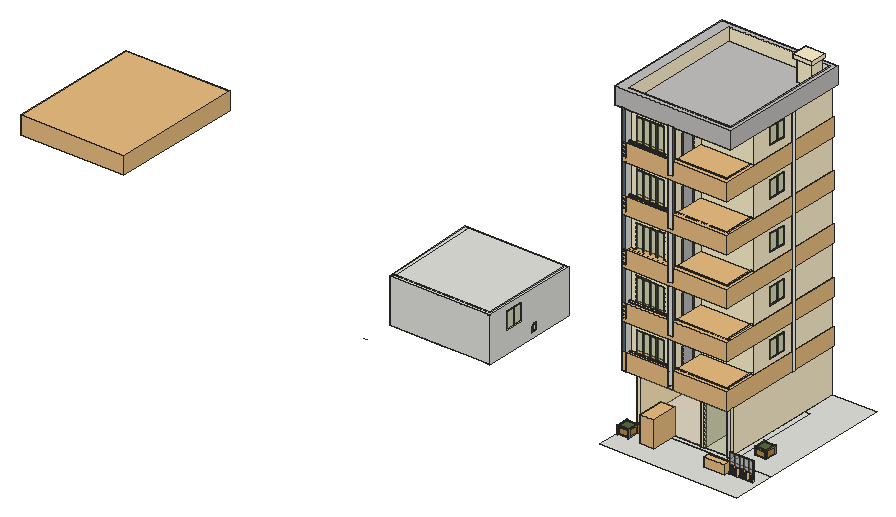
# SketchUp Ruby script. Lengths in inches.
U = 1.inch
M = Sketchup.active_model
def pt(a) = Geom::Point3d.new(a.map { |v| v * U })
def face(e, loops, mat)
  f = e.add_face(loops[0].map { |a| pt(a) })
  loops[1..].each { |l| e.add_face(l.map { |a| pt(a) }).erase! }
  f.material = f.back_material = mat if mat
  f
end
# faces: each face lists its corners as indices into pts; further lists are holes
def faces(e, pts, list, mat = nil) = list.each { |f| face(e, (f[0].is_a?(Array) ? f : [f]).map { |l| l.map { |i| pts[i] } }, mat) }
# xy, xz, yz: faces in a plane at the given z, y or x. An outline is a flat list of corners, or four numbers for a rectangle; further outlines are holes
def ring(l) = l.size == 4 ? [[l[0], l[1]], [l[2], l[1]], [l[2], l[3]], [l[0], l[3]]] : l.each_slice(2).to_a
def flat(e, list, mat, &to3) = list.each { |f| face(e, (f[0].is_a?(Array) ? f : [f]).map { |l| ring(l).map { |u, v| to3.(u, v) } }, mat) }
def xy(e, z, list, mat = nil) = flat(e, list, mat) { |x, y| [x, y, z] }
def xz(e, y, list, mat = nil) = flat(e, list, mat) { |x, z| [x, y, z] }
def yz(e, x, list, mat = nil) = flat(e, list, mat) { |y, z| [x, y, z] }
def lines(e, pts, list) = list.each { |a, b| e.add_line(pt(pts[a]), pt(pts[b])) }
# prism: a flat outline (further loops are holes) pulled along v
def prism(e, loops, v, mat = nil)
  f = face(e, loops, mat); d = Geom::Vector3d.new(v.map { |x| x * U })
  f.pushpull(f.normal.samedirection?(d) ? d.length : -d.length)
end
def box(e, o, s, mat = nil) = prism(e, [[o, [o[0] + s[0], o[1], o[2]], [o[0] + s[0], o[1] + s[1], o[2]], [o[0], o[1] + s[1], o[2]]]], [0, 0, s[2]], mat)
def at(x, y, z, deg = 0) = Geom::Transformation.translation(pt([x, y, z])) * Geom::Transformation.rotation(ORIGIN, Z_AXIS, deg.degrees)
def axes(o, x, y, z) = Geom::Transformation.new([*x, 0, *y, 0, *z, 0, *pt(o).to_a, 1])
def part(name) = M.definitions.add(name)
# library, detail: a bought-in or finely detailed component or shape, given as its bounding box
def library(name, o, s) = part(name).tap { |d| box(d.entities, o, s) }
def detail(e, o, s) = box(e.add_group.entities, o, s)
def put(e, d, t, mat = nil) = e.add_instance(d, t).tap { |i| i.material = mat if mat }
def group(e, t, mat = nil) = e.add_group.tap { |g| g.transformation = t; g.material = mat if mat }.entities
root = M.entities
M.materials.add("!长灌木1").color = [90, 107, 61]
M.materials.add("Carpet_01_1K").color = [196, 195, 193]
M.materials.add("D01_Frost_White").color = [255, 242, 206]
M.materials.add("Denim_03_1K").color = [93, 106, 119]
M.materials.add("Glass_Basic_01").color = [179, 186, 71]
M.materials["Glass_Basic_01"].alpha = 0.25
M.materials.add("Glass_Basic_1").color = [255, 210, 130]
M.materials["Glass_Basic_1"].alpha = 0.25
M.materials.add("Glass_Mirror_01").color = [185, 185, 185]
M.materials.add("M00_Soft_Cloud").color = [255, 255, 255]
M.materials.add("Material20").color = [184, 138, 65]
M.materials.add("Material48").color = [126, 124, 110]
M.materials.add("Material__1").color = [95, 70, 46]
M.materials.add("Wood_Planks_01_1K").color = [69, 67, 63]
M.materials.add("[Color M00]").color = [255, 255, 255]
M.materials.add("[Translucent Glass Gray]").color = [128, 128, 128]
M.materials["[Translucent Glass Gray]"].alpha = 0.29
M.materials.add("homalw").color = [47, 64, 22]
M.materials.add("palmleaf1").color = [111, 131, 65]
c1 = library("Balcony with railing",[0,-15.52,0],[286.53,362.52,46.98])
c2 = part("Building bay")
xy(c2.entities,0,[[0,-15.52,12,0],[125.84,-15.52,138,0],[9,9,129,80],[9,89,273,338]])
xy(c2.entities,16.02,[[273,223.5625,282,234.47]])
xy(c2.entities,34.07,[[273,223.5625,282,234.47]])
xy(c2.entities,120,[[0,-15.52,9,347],[9,-15.52,12,-15.52,12,0,125.84,0,125.84,-15.52,138,-15.52,138,80.06,282,80.06,282,347,9,347,9,338,273,338,273,89,9,89,9,80,129,80,129,9,9,9],[9,89,273,338]])
xy(c2.entities,120,[[9,9,129,80]],"Denim_03_1K")
xz(c2.entities,-15.52,[[125.84,0,138,120]])
xz(c2.entities,-15.52,[[0,0,12,120]],"Denim_03_1K")
xz(c2.entities,0,[[[12,0,125.84,120],[26.96,12.98,106.4,103.84]]],"D01_Frost_White")
xz(c2.entities,0,[[29.96,15.98,45.32,100.84],[48.32,15.98,63.68,100.84],[66.68,15.98,82.04,100.84],[85.04,15.98,103.4,100.84]],"Glass_Basic_01")
xz(c2.entities,0,[[[26.96,12.98,106.4,103.84],[85.04,15.98,103.4,100.84],[48.32,15.98,63.68,100.84],[66.68,15.98,82.04,100.84],[29.96,15.98,45.32,100.84]]],"Wood_Planks_01_1K")
xz(c2.entities,9,[[9,0,129,120]])
xz(c2.entities,80,[[9,0,129,120]])
xz(c2.entities,80.06,[[138,0,282,120]],"D01_Frost_White")
xz(c2.entities,89,[[9,0,273,120]])
xz(c2.entities,223.5625,[[273,16.02,282,34.07]])
xz(c2.entities,234.47,[[273,16.02,282,34.07]])
xz(c2.entities,338,[[9,0,273,120]])
xz(c2.entities,347,[[0,0,282,120]])
yz(c2.entities,0,[[-15.52,0,347,120]],"D01_Frost_White")
yz(c2.entities,9,[[9,0,80,120],[89,0,338,120]])
yz(c2.entities,12,[[-15.52,0,0,120]])
yz(c2.entities,125.84,[[-15.52,0,0,120]])
yz(c2.entities,129,[[9,0,80,120]])
yz(c2.entities,138,[[-7.18,10,-7.09,120]])
yz(c2.entities,138,[[[-15.52,0,80.06,0,80.06,120,-7.09,120,-7.09,10,-15.52,10],[17.75,12.24,56.41,97.36]]],"D01_Frost_White")
yz(c2.entities,138,[[-15.52,10,-7.18,120]],"Denim_03_1K")
yz(c2.entities,138,[[20.75,15.24,53.41,94.36]],"Glass_Mirror_01")
yz(c2.entities,138,[[[17.75,12.24,56.41,97.36],[20.75,15.24,53.41,94.36]]],"Wood_Planks_01_1K")
yz(c2.entities,273,[[[89,0,338,120],[223.5625,16.02,234.47,34.07]]])
yz(c2.entities,282,[[[80.06,0,347,120],[133.09,55.97,187.08,106.98],[222.16,14.62,235.875,35.48]]],"D01_Frost_White")
yz(c2.entities,282,[[136.83,59.71,160.08,103.24],[163.08,59.71,183.34,103.24]],"Glass_Basic_01")
yz(c2.entities,282,[[[222.16,14.62,235.875,35.48],[223.5625,16.02,234.47,34.07]],[[133.09,55.97,187.08,106.98],[136.83,59.71,183.34,103.24]],[160.08,59.71,163.08,103.24]],"Wood_Planks_01_1K")
c3 = part("Flat roof assembly")
xy(c3.entities,-639.97,[[282,205.21,288.51,211.41]])
xy(c3.entities,-6.48,[[158.77,-7.18,158.77,211.41,282,211.41,282,205.21,288.51,205.21,288.51,-7.18],[282,211.41,282,211.54,293.15,211.41]])
xy(c3.entities,0,[[[-17.96,-15,297.5,347],[158.77,-7.18,288.51,211.41]]])
xy(c3.entities,10,[[[11.4,-3.6,286.1,335.6],[232.625,289.57,272.46,324.45]]],"Carpet_01_1K")
xy(c3.entities,46,[[[-17.96,-15,297.5,347],[11.4,-3.6,286.1,335.6]]],"Carpet_01_1K")
xy(c3.entities,66.73,[[[224.49,284,277.47,329.34],[232.625,289.57,272.46,324.45]],[232.625,289.57,272.46,324.45]])
xy(c3.entities,76.73,[[224.49,284,277.47,329.34]])
xz(c3.entities,-15,[[-17.96,0,297.5,46]],"Carpet_01_1K")
xz(c3.entities,-7.18,[[158.77,-6.48,288.51,0]])
xz(c3.entities,-3.6,[[11.4,10,12,46]])
xz(c3.entities,-3.6,[[12,10,125.84,46],[125.84,10,138,46],[138,10,286.1,46]],"Carpet_01_1K")
xz(c3.entities,205.21,[[282,-639.97,288.51,-6.48]])
xz(c3.entities,211.41,[[282,-639.97,288.51,-6.48],[158.77,-6.48,288.51,0]])
xz(c3.entities,284,[[224.49,66.73,277.47,76.73]])
xz(c3.entities,289.57,[[232.625,10,272.46,66.73]])
xz(c3.entities,324.45,[[232.625,10,272.46,66.73]])
xz(c3.entities,329.34,[[224.49,66.73,277.47,76.73]])
xz(c3.entities,335.6,[[11.4,10,286.1,46]])
xz(c3.entities,347,[[-17.96,0,297.5,46]],"Carpet_01_1K")
yz(c3.entities,-17.96,[[-15,0,347,46]],"Carpet_01_1K")
yz(c3.entities,11.4,[[-3.6,10,335.6,46]])
yz(c3.entities,158.77,[[-7.18,-6.48,211.41,0]])
yz(c3.entities,224.49,[[284,66.73,329.34,76.73]])
yz(c3.entities,232.625,[[289.57,10,324.45,66.73]])
yz(c3.entities,272.46,[[289.57,10,324.45,66.73]])
yz(c3.entities,277.47,[[284,66.73,329.34,76.73]])
yz(c3.entities,282,[[205.21,-639.97,211.41,-6.48]])
yz(c3.entities,286.1,[[-3.6,10,335.6,46]],"Carpet_01_1K")
yz(c3.entities,288.51,[[205.21,-639.97,211.41,-639.97,211.41,0,-7.18,0,-7.18,-6.48,205.21,-6.48]],"M00_Soft_Cloud")
yz(c3.entities,297.5,[[-15,0,347,46]],"Carpet_01_1K")
c4 = library("Balcony railing",[0,-12,0],[282,359,46.98])
c5 = part("组\#1")
xy(c5.entities,0,[[0,0,2.36,2.36],[29.92,0,32.28,2.36],[0,29.92,2.36,32.28],[29.92,29.92,32.28,32.28]],"Material48")
xy(c5.entities,1.57,[[2.36,0.39,2.36,2.36,0.39,2.36,0.39,29.92,2.36,29.92,2.36,31.89,29.92,31.89,29.92,29.92,31.89,29.92,31.89,2.36,29.92,2.36,29.92,0.39]],"Material48")
xy(c5.entities,2.76,[[3.54,0.39,28.74,1.57],[0.39,3.54,1.57,28.74],[30.71,3.54,31.89,28.74],[3.54,30.71,28.74,31.89]],"Material20")
xy(c5.entities,20.08,[[3.54,0.39,28.74,1.57],[0.39,3.54,1.57,28.74],[30.71,3.54,31.89,28.74],[3.54,30.71,28.74,31.89]],"Material20")
xy(c5.entities,21.0625,[[2.36,2.36,29.92,29.92]],"!长灌木1")
xy(c5.entities,21.26,[[2.36,0.39,29.92,2.36],[0.39,2.36,2.36,29.92],[29.92,2.36,31.89,29.92],[2.36,29.92,29.92,31.89]],"Material20")
xy(c5.entities,21.38,[[2.36,2.36,29.92,29.92]],"!长灌木1")
xy(c5.entities,22.83,[[0,0,2.36,2.36],[29.92,0,32.28,2.36],[0,29.92,2.36,32.28],[29.92,29.92,32.28,32.28]],"Material20")
xz(c5.entities,0,[[0,0,2.36,22.83],[29.92,0,32.28,22.83]],"Material20")
xz(c5.entities,0.39,[[[2.36,1.57,29.92,21.26],[3.54,2.76,28.74,20.08]]],"Material20")
xz(c5.entities,1.57,[[3.54,2.76,28.74,20.08]],"Material20")
xz(c5.entities,2.36,[[2.36,21.0625,29.92,21.38],[2.36,21.26,29.92,23.43]],"!长灌木1")
xz(c5.entities,2.36,[[0,0,0,22.83,2.36,22.83,2.36,21.26,0.39,21.26,0.39,1.57,2.36,1.57,2.36,0],[29.92,0,29.92,1.57,31.89,1.57,31.89,21.26,29.92,21.26,29.92,22.83,32.28,22.83,32.28,0]],"Material20")
xz(c5.entities,3.54,[[0.39,2.76,1.57,20.08],[30.71,2.76,31.89,20.08]],"Material20")
xz(c5.entities,28.74,[[0.39,2.76,1.57,20.08],[30.71,2.76,31.89,20.08]],"Material20")
xz(c5.entities,29.92,[[2.36,21.0625,29.92,21.38],[2.36,21.26,29.92,23.43]],"!长灌木1")
xz(c5.entities,29.92,[[0,0,2.36,0,2.36,1.57,0.39,1.57,0.39,22.83,0,22.83],[29.92,0,32.28,0,32.28,22.83,31.89,22.83,31.89,1.57,29.92,1.57],[0.39,21.26,2.36,22.83],[29.92,21.26,31.89,22.83]],"Material20")
xz(c5.entities,30.71,[[3.54,2.76,28.74,20.08]],"Material20")
xz(c5.entities,31.89,[[[2.36,1.57,29.92,21.26],[3.54,2.76,28.74,20.08]]],"Material20")
xz(c5.entities,32.28,[[0,0,2.36,22.83],[29.92,0,32.28,22.83]],"Material20")
yz(c5.entities,0,[[0,0,2.36,22.83],[29.92,0,32.28,22.83]],"Material20")
yz(c5.entities,0.39,[[[2.36,1.57,29.92,21.26],[3.54,2.76,28.74,20.08]]],"Material20")
yz(c5.entities,1.57,[[3.54,2.76,28.74,20.08]],"Material20")
yz(c5.entities,2.36,[[0,0,2.36,0,2.36,1.57,0.39,1.57,0.39,22.83,0,22.83]])
yz(c5.entities,2.36,[[2.36,21.0625,29.92,21.38],[2.36,21.26,29.92,23.43]],"!长灌木1")
yz(c5.entities,2.36,[[29.92,0,32.28,0,32.28,22.83,29.92,22.83,29.92,21.26,31.89,21.26,31.89,1.57,29.92,1.57],[0.39,21.26,2.36,22.83]],"Material20")
yz(c5.entities,3.54,[[0.39,2.76,1.57,20.08],[30.71,2.76,31.89,20.08]],"Material20")
yz(c5.entities,28.74,[[0.39,2.76,1.57,20.08],[30.71,2.76,31.89,20.08]],"Material20")
yz(c5.entities,29.92,[[2.36,21.0625,29.92,21.38],[2.36,21.26,29.92,23.43]],"!长灌木1")
yz(c5.entities,29.92,[[0,0,0,22.83,2.36,22.83,2.36,21.26,0.39,21.26,0.39,1.57,2.36,1.57,2.36,0],[29.92,0,29.92,1.57,31.89,1.57,31.89,21.26,29.92,21.26,29.92,22.83,32.28,22.83,32.28,0]],"Material20")
yz(c5.entities,30.71,[[3.54,2.76,28.74,20.08]],"Material20")
yz(c5.entities,31.89,[[[2.36,1.57,29.92,21.26],[3.54,2.76,28.74,20.08]]],"Material20")
yz(c5.entities,32.28,[[0,0,2.36,22.83],[29.92,0,32.28,22.83]],"Material20")
c6 = part("组\#2")
put(c6.entities,c5,at(24.1,23.99,0))
c7 = part("Tree in planter")
put(c7.entities,c6,at(-24.1,-23.99,-1.57))
c8 = library("Planted timber trough",[0,0,0],[56.02,15.3,25.28])
c9 = library("Group_2",[-1.28,-0.39,0],[21.22,20.51,48.44])
c10 = library("Areca palm plant",[0,0,0],[49.1,36.6,54.46])
c11 = part("W1")
xy(c11.entities,15,[[0,0,2,198]])
xy(c11.entities,102.0625,[[0,0,2,198]],"[Color M00]")
xz(c11.entities,0,[[0,15,2,102.0625]],"[Color M00]")
xz(c11.entities,198,[[0,15,2,102.0625]])
yz(c11.entities,0,[[0.84,16,39.43,101.0625],[40.28,16,78.87,101.0625],[79.71,16,118.3,101.0625],[119.14,16,157.73,101.0625],[158.58,16,197.16,101.0625]])
yz(c11.entities,0,[[[0,15,198,102.0625],[0.84,16,197.16,101.0625]],[39.43,16,40.28,101.0625],[78.87,16,79.71,101.0625],[118.3,16,119.14,101.0625],[157.73,16,158.58,101.0625]],"[Color M00]")
yz(c11.entities,2,[[0.84,16,39.43,101.0625],[40.28,16,78.87,101.0625],[79.71,16,118.3,101.0625],[119.14,16,157.73,101.0625],[158.58,16,197.16,101.0625]])
yz(c11.entities,2,[[[0,15,198,102.0625],[0.84,16,197.16,101.0625]],[39.43,16,40.28,101.0625],[78.87,16,79.71,101.0625],[118.3,16,119.14,101.0625],[157.73,16,158.58,101.0625]],"[Color M00]")
c12 = part("Leaf \#1")
xy(c12.entities,0,[[-7.96,70.18,-15.37,80.78,-8.51,79.39]],"homalw")
p = [[0,3.11,-13.12],[-2.47,2.5625,-12.61],[-0.33,11.57,-7.99],[2.47,2.5625,-12.61],[0.85,11.07,-7.46],[-1.5,10.97,-7.51],
  [-1.3,12.65,-6.5],[0.75,12.74,-6.45],[-0.28,13.24,-6.98],[-0.52,17.92,-5.25],[0.26,22.09,-2.99],[-2.03,21.56,-3.1875],
  [-0.88,22.37,-3.6],[-7.14,103.99,-5.5],[-9.49,101.08,-4.85],[-14.75,100.84,-3.42],[-8.43,101.53,-4.95],[-9.71,91.2,-2.64],
  [-6.77,97.58,-4.07],[-9.11,85.3,-1.32],[-1.78,90.91,-2.58],[-1.73,26.48,-2.37],[-19.59,96.71,-2.34],[-6.15,22.74,-2.99],
  [3.7,24.59,-2.68],[-10.51,27.34,-0.03],[6.46,30.29,-1.74],[-8.51,79.39,0],[2.35,82.65,1.85],[-2.58,31.13,-1.6],
  [8.32,35.3,1.04],[-22.78,91.25,-1.85],[-15.37,80.78,0],[-23.64,83.39,1.26],[-18.25,46.35,2.71],[-4.82,40.8125,0],
  [10.88,46.34,4.1875],[-5.85,48.04,0],[9.36,55.76,0],[-20.59,57.25,0.91],[-24.7,67.99,2.4],[-7.2,57.46,0],
  [8.22,62.39,2.8],[-7.41,60.98,0],[1.46,71.64,1.73],[-25.52,72,2.4],[-7.96,70.18,0],[-24.41,76.18,0],
  [-23.875,81.13,1.26],[3.03,76.55,1.0625]]
faces(c12.entities,p,[[0,1,2],[3,0,4],[2,4,0],[5,2,1],[5,6,2],[4,2,7],[8,2,6],[8,7,2],
  [6,9,8],[7,8,9,10],[9,6,11,12],[13,14,15],[13,16,14],[10,9,12],[17,14,16,18],[17,15,14],
  [17,18,19],[20,19,18],[11,21,12],[10,12,21],[22,15,19],[17,19,15],[23,21,11],[24,10,21],
  [23,25,21],[24,21,26],[19,20,27],[28,27,20],[25,29,21],[30,21,29],[26,21,30],[22,19,31],
  [27,31,19],[31,27,32],[31,32,33],[25,34,29],[35,29,34],[35,36,29],[30,29,36],[35,34,37],
  [35,37,36],[38,36,37],[39,37,34],[39,40,37],[41,37,40],[42,37,41],[42,38,37],[41,40,43],
  [43,44,41],[42,41,44],[43,45,46],[45,43,40],[43,46,44],[45,47,46],[48,46,47],[48,33,46],
  [32,46,33],[27,44,46],[44,27,49],[28,49,27]],"homalw")
c13 = part("Leaf \#2")
xy(c13.entities,0,[[-7.96,70.18,-15.37,80.78,-8.51,79.39]],"homalw")
p = [[0,3.11,-13.12],[-2.47,2.5625,-12.61],[-0.33,11.57,-7.99],[2.47,2.5625,-12.61],[0.85,11.07,-7.46],[-1.5,10.97,-7.51],
  [-1.3,12.65,-6.5],[0.75,12.74,-6.45],[-0.28,13.24,-6.98],[-0.52,17.92,-5.25],[0.26,22.09,-2.99],[-2.03,21.56,-3.1875],
  [-0.88,22.37,-3.6],[-7.14,103.99,-5.5],[-9.49,101.08,-4.85],[-14.75,100.84,-3.42],[-8.43,101.53,-4.95],[-9.71,91.2,-2.64],
  [-6.77,97.58,-4.07],[-9.11,85.3,-1.32],[-1.78,90.91,-2.58],[-1.73,26.48,-2.37],[-19.59,96.71,-2.34],[-6.15,22.74,-2.99],
  [3.7,24.59,-2.68],[-10.51,27.34,-0.03],[6.46,30.29,-1.74],[-8.51,79.39,0],[2.35,82.65,1.85],[-2.58,31.13,-1.6],
  [8.32,35.3,1.04],[-22.78,91.25,-1.85],[-15.37,80.78,0],[-23.64,83.39,1.26],[-18.25,46.35,2.71],[-4.82,40.8125,0],
  [10.88,46.34,4.1875],[-5.85,48.04,0],[9.36,55.76,0],[-20.59,57.25,0.91],[-24.7,67.99,2.4],[-7.2,57.46,0],
  [8.22,62.39,2.8],[-7.41,60.98,0],[1.46,71.64,1.73],[-25.52,72,2.4],[-7.96,70.18,0],[-24.41,76.18,0],
  [-23.875,81.13,1.26],[3.03,76.55,1.0625]]
faces(c13.entities,p,[[0,1,2],[3,0,4],[2,4,0],[5,2,1],[5,6,2],[4,2,7],[8,2,6],[8,7,2],
  [6,9,8],[7,8,9,10],[9,6,11,12],[13,14,15],[13,16,14],[10,9,12],[17,14,16,18],[17,15,14],
  [17,18,19],[20,19,18],[11,21,12],[10,12,21],[22,15,19],[17,19,15],[23,21,11],[24,10,21],
  [23,25,21],[24,21,26],[19,20,27],[28,27,20],[25,29,21],[30,21,29],[26,21,30],[22,19,31],
  [27,31,19],[31,27,32],[31,32,33],[25,34,29],[35,29,34],[35,36,29],[30,29,36],[35,34,37],
  [35,37,36],[38,36,37],[39,37,34],[39,40,37],[41,37,40],[42,37,41],[42,38,37],[41,40,43],
  [43,44,41],[42,41,44],[43,45,46],[45,43,40],[43,46,44],[45,47,46],[48,46,47],[48,33,46],
  [32,46,33],[27,44,46],[44,27,49],[28,49,27]],"homalw")
c14 = part("Leaf \#8")
p = [[0,3.11,-17.57],[-2.47,2.5625,-17.06],[-0.33,11.57,-12.44],[2.47,2.5625,-17.06],[0.85,11.07,-11.9],[-1.5,10.97,-11.96],
  [-1.3,12.65,-10.95],[0.75,12.74,-10.9],[-0.28,13.24,-11.43],[-0.52,17.92,-9.7],[0.26,22.09,-7.4375],[-2.03,21.56,-7.64],
  [-0.88,22.37,-8.05],[-1.73,26.48,-6.82],[-6.15,22.74,-2.99],[3.7,24.59,-2.68],[-9.71,91.2,-7.09],[-9.11,85.3,-5.77],
  [-14.75,100.84,-3.42],[-6.77,97.58,-4.07],[-9.49,101.08,-5.6],[-10.51,27.34,-0.03],[6.46,30.29,-1.74],[-2.58,31.13,-6.05],
  [8.32,35.3,1.04],[-18.25,46.35,2.71],[-4.82,40.8125,-4.45],[10.88,46.34,4.1875],[-8.51,79.39,-4.45],[-22.78,91.25,-1.85],
  [-1.78,90.91,-2.58],[-19.59,96.71,-2.34],[-8.43,101.53,-4.95],[-7.14,103.99,-5.5],[-5.85,48.04,-4.45],[9.36,55.76,0],
  [-20.59,57.25,0.91],[-24.7,67.99,2.4],[-7.2,57.46,-4.45],[8.22,62.39,2.8],[-7.41,60.98,-4.45],[1.46,71.64,1.73],
  [-25.52,72,2.4],[-7.96,70.18,-4.45],[-24.41,76.18,0],[-23.875,81.13,1.26],[-23.64,83.39,1.26],[-15.37,80.78,0],
  [3.03,76.55,1.0625],[2.35,82.65,1.85]]
faces(c14.entities,p,[[0,1,2],[3,0,4],[2,4,0],[5,2,1],[5,6,2],[4,2,7],[8,2,6],[8,7,2],
  [6,9,8],[7,8,9,10],[9,6,11,12],[10,9,12],[11,13,12],[10,12,13],[14,13,11],[15,10,13],
  [16,17,18],[16,19,17],[16,18,20],[19,16,20],[14,21,13],[15,13,22],[21,23,13],[24,13,23],
  [22,13,24],[21,25,23],[26,23,25],[26,27,23],[24,23,27],[28,29,17],[17,30,28],[31,17,29],
  [31,18,17],[30,17,19],[20,32,19],[33,20,18],[33,32,20],[26,25,34],[26,34,27],[35,27,34],
  [36,34,25],[36,37,34],[38,34,37],[39,34,38],[39,35,34],[38,37,40],[40,41,38],[39,38,41],
  [40,42,43],[42,40,37],[40,43,41],[42,44,43],[45,43,44],[45,46,43],[47,43,46],[43,47,28],
  [28,41,43],[41,28,48],[49,48,28],[29,28,47],[49,28,30],[29,47,46]],"homalw")
c15 = part("Leaf \#4")
xy(c15.entities,0,[[-7.96,70.18,-15.37,80.78,-8.51,79.39]],"homalw")
p = [[0,3.11,-13.12],[-2.47,2.5625,-12.61],[-0.33,11.57,-7.99],[2.47,2.5625,-12.61],[0.85,11.07,-7.46],[-1.5,10.97,-7.51],
  [-1.3,12.65,-6.5],[0.75,12.74,-6.45],[-0.28,13.24,-6.98],[-0.52,17.92,-5.25],[0.26,22.09,-2.99],[-2.03,21.56,-3.1875],
  [-0.88,22.37,-3.6],[-7.14,103.99,-5.5],[-9.49,101.08,-4.85],[-14.75,100.84,-3.42],[-8.43,101.53,-4.95],[-9.71,91.2,-2.64],
  [-6.77,97.58,-4.07],[-9.11,85.3,-1.32],[-1.78,90.91,-2.58],[-1.73,26.48,-2.37],[-19.59,96.71,-2.34],[-6.15,22.74,-2.99],
  [3.7,24.59,-2.68],[-10.51,27.34,-0.03],[6.46,30.29,-1.74],[-8.51,79.39,0],[2.35,82.65,1.85],[-2.58,31.13,-1.6],
  [8.32,35.3,1.04],[-22.78,91.25,-1.85],[-15.37,80.78,0],[-23.64,83.39,1.26],[-18.25,46.35,2.71],[-4.82,40.8125,0],
  [10.88,46.34,4.1875],[-5.85,48.04,0],[9.36,55.76,0],[-20.59,57.25,0.91],[-24.7,67.99,2.4],[-7.2,57.46,0],
  [8.22,62.39,2.8],[-7.41,60.98,0],[1.46,71.64,1.73],[-25.52,72,2.4],[-7.96,70.18,0],[-24.41,76.18,0],
  [-23.875,81.13,1.26],[3.03,76.55,1.0625]]
faces(c15.entities,p,[[0,1,2],[3,0,4],[2,4,0],[5,2,1],[5,6,2],[4,2,7],[8,2,6],[8,7,2],
  [6,9,8],[7,8,9,10],[9,6,11,12],[13,14,15],[13,16,14],[10,9,12],[17,14,16,18],[17,15,14],
  [17,18,19],[20,19,18],[11,21,12],[10,12,21],[22,15,19],[17,19,15],[23,21,11],[24,10,21],
  [23,25,21],[24,21,26],[19,20,27],[28,27,20],[25,29,21],[30,21,29],[26,21,30],[22,19,31],
  [27,31,19],[31,27,32],[31,32,33],[25,34,29],[35,29,34],[35,36,29],[30,29,36],[35,34,37],
  [35,37,36],[38,36,37],[39,37,34],[39,40,37],[41,37,40],[42,37,41],[42,38,37],[41,40,43],
  [43,44,41],[42,41,44],[43,45,46],[45,43,40],[43,46,44],[45,47,46],[48,46,47],[48,33,46],
  [32,46,33],[27,44,46],[44,27,49],[28,49,27]],"homalw")
c16 = part("Group\#74")
put(c16.entities,c12,axes([-2.14,10.62,47.33],[-0.95106,-0.30902,0],[0.16301,-0.50171,1.04433],[-0.27582,0.8489,0.45088]))
put(c16.entities,c13,axes([-4.29,11.23,21.36],[-0.87377,-0.48634,0],[0.33168,-0.59591,0.73135],[-0.35568,0.63904,0.682]))
put(c16.entities,c12,axes([0.5625,10.16,42.52],[1.1881,-0.15086,-0.19526],[0.05565,-0.5973,0.80009],[0.19558,0.79233,0.5779]))
put(c16.entities,c12,axes([4.1,3.11,43.35],[-0.41921,0.53472,0.02711],[-0.3495,-0.29938,0.50061],[0.4056,0.29469,0.4594]))
put(c16.entities,c13,axes([-2.57,-6.41,36.43],[0.53452,-0.58924,-0.60587],[0.84017,0.2927,0.45656],[-0.09168,-0.75307,0.65152]))
put(c16.entities,c12,axes([-5.26,9.47,47.75],[-0.43808,-0.60296,0],[0.36477,-0.26502,0.89259],[-0.72212,0.52465,0.45088]))
put(c16.entities,c14,axes([6.53,-10.1875,67.1],[-0.90669,-0.3353,-0.25591],[-0.33003,0.18612,0.92544],[0.26267,-0.92355,0.27941]))
put(c16.entities,c12,axes([5.77,-7.56,44.11],[0.8933,-0.05321,0.44629],[-0.40292,0.34518,0.84765],[-0.19916,-0.93703,0.28691]))
put(c16.entities,c13,axes([-5.05,-10.15,21.36],[0.95106,-0.30902,0],[0.21075,0.64862,0.73135],[-0.226,-0.69556,0.682]))
put(c16.entities,c12,axes([12.18,-10.02,43.56],[0.58779,0.80902,0],[-0.41219,0.29947,1.00862],[1.44423,-1.0493,0.90176]))
put(c16.entities,c12,axes([-7.64,-4.83,47.75],[0.58779,-0.80902,0],[0.36477,0.26502,0.89259],[-0.72212,-0.52465,0.45088]))
put(c16.entities,c13,axes([13.57,-1.5625,21.36],[0,1,0],[-0.682,0,0.73135],[0.73135,0,0.682]))
put(c16.entities,c13,axes([1.77,-4.48,63.77],[-0.82031,0.42803,0.37932],[0.41775,0.36976,0.48618],[-0.09168,-0.75307,0.65152]))
put(c16.entities,c15,axes([-9.15,4.95,23.72],[-0.58779,-0.80902,0],[0.67618,-0.49128,0.54902],[-0.44417,0.32271,0.83581]))
put(c16.entities,c15,axes([3.34,7.33,23.69],[-0.95106,0.30902,0],[-0.25828,-0.7949,0.54902],[0.16966,0.52215,0.83581]))
put(c16.entities,c15,axes([6.45,-6.01,23.69],[0.58779,0.80902,0],[-0.67618,0.49128,0.54902],[0.44417,-0.32271,0.83581]))
put(c16.entities,c15,axes([1.375,-7.81,23.69],[0.95106,0.30902,0],[-0.25828,0.7949,0.54902],[0.16966,-0.52215,0.83581]))
put(c16.entities,c13,axes([2.63,-11.68,6.71],[0.95106,0.30902,0],[-0.21075,0.64862,0.73135],[0.226,-0.69556,0.682]))
g1 = group(c16.entities,at(-3.46,-3.57,-0.02),"palmleaf1")
xy(g1,0,[[4.54,0,0.96,0.96,0,4.53,2.62,7.15,6.19,6.2,7.16,2.62]])
xy(g1,55.42,[[4.39,0.55,6.6,2.77,5.79,5.79,2.77,6.6,0.55,4.38,1.37,1.36]])
p = [[4.54,0,0],[4.39,0.55,55.42],[1.37,1.36,55.42],[0.96,0.96,0],[7.16,2.62,0],[6.6,2.77,55.42],
  [0.55,4.38,55.42],[0,4.53,0],[6.19,6.2,0],[5.79,5.79,55.42],[2.77,6.6,55.42],[2.62,7.15,0]]
faces(g1,p,[[0,1,2,3],[0,4,5,1],[3,2,6,7],[4,8,9,5],[6,10,11,7],[11,10,9,8]])
c17 = library("Group20\#1",[-20.81,-17.08,3.79],[39.86,39.43,37.51])
c18 = library("Group\#130",[-7.34,-1.2,0],[38.67,35.81,49.04])
c19 = library("Group38\#2",[14.01,28.44,-23.43],[18.58,18.32,38.89])
c20 = part("PLANTS (1)")
put(c20.entities,c10,axes([38.49,169.84,6.02],[0.45017,-0.56191,0],[0.66137,0.52986,0],[0,0,0.72]))
put(c20.entities,c10,axes([38.49,68.02,6.02],[0.45017,-0.56191,0],[0.66137,0.52986,0],[0,0,0.72]))
put(c20.entities,c11,axes([76.68,11.43,-0.0625],[1,0,0],[0,1.18586,0],[0,0,1]),"[Translucent Glass Gray]")
put(c20.entities,c16,axes([59.61,184.54,5.99],[-0.04961,-0.08593,0],[0.08593,-0.04961,0],[0,0,0.10522]))
put(c20.entities,c16,axes([59.61,204.61,5.99],[-0.04961,-0.08593,0],[0.08593,-0.04961,0],[0,0,0.10522]))
put(c20.entities,c16,axes([59.61,157.29,5.99],[-0.04961,-0.08593,0],[0.08593,-0.04961,0],[0,0,0.10522]))
put(c20.entities,c17,axes([63.65,91.4,4.71],[0,0.85,0],[-0.85,0,0],[0,0,0.85]))
put(c20.entities,c18,axes([69.62,101.34,7.93],[0,0.79,0],[-0.79,0,0],[0,0,0.79]))
put(c20.entities,c19,axes([40.58,10.27,28.11],[0.8848,0,0],[0,0.94674,0],[0,0,0.85826]))
put(c20.entities,c16,axes([59.61,55.48,5.99],[-0.04961,-0.08593,0],[0.08593,-0.04961,0],[0,0,0.10522]))
put(c20.entities,c16,axes([59.61,82.73,5.99],[-0.04961,-0.08593,0],[0.08593,-0.04961,0],[0,0,0.10522]))
put(c20.entities,c16,axes([61.875,132.66,6.01],[-0.08133,-0.14087,0],[0.14087,-0.08133,0],[0,0,0.1725]))
put(c20.entities,c16,axes([59.61,102.79,5.99],[-0.04961,-0.08593,0],[0.08593,-0.04961,0],[0,0,0.10522]))
put(c20.entities,c16,axes([61.875,27.22,6.01],[-0.08133,-0.14087,0],[0.14087,-0.08133,0],[0,0,0.1725]))
put(c20.entities,c16,axes([61.875,234.47,6.01],[-0.08133,-0.14087,0],[0.14087,-0.08133,0],[0,0,0.1725]))
put(c20.entities,c18,axes([69.62,203.15,7.93],[0,0.79,0],[-0.79,0,0],[0,0,0.79]))
put(c20.entities,c17,axes([63.65,193.21,4.71],[0,0.85,0],[-0.85,0,0],[0,0,0.85]))
put(c20.entities,c19,axes([40.58,112.08,28.11],[0.8848,0,0],[0,0.94674,0],[0,0,0.85826]))
g2 = group(c20.entities,at(44.68,11.43,-0.0625))
xy(g2,0,[[0,0,6,234.8],[30,0,36,234.8]])
xy(g2,3,[[6,0,30,234.8]])
xy(g2,7,[[6,5,30,229.8]],"Material__1")
xy(g2,15,[[[0,0,36,234.8],[6,5,30,229.8]]])
xz(g2,0,[[0,0,6,0,6,3,30,3,30,0,36,0,36,15,0,15]])
xz(g2,5,[[6,7,30,15]])
xz(g2,229.8,[[6,7,30,15]])
xz(g2,234.8,[[0,0,0,15,36,15,36,0,30,0,30,3,6,3,6,0]])
yz(g2,0,[[0,0,234.8,15]])
yz(g2,6,[[0,0,234.8,3],[5,7,229.8,15]])
yz(g2,30,[[0,0,234.8,3],[5,7,229.8,15]])
yz(g2,36,[[0,0,234.8,15]])
prism(root,[[[919.67,123.27,795.09],[919.67,125.89,795.09],[1055.6,125.89,795.09],[1055.6,206.86,795.09],[1057.43,206.86,795.09],[1057.43,123.27,795.09]]],[0,0,1.89])
box(root,[793.67,118.83,407.88],[113.63,4.95,2.51])
box(root,[792.82,119.01,285.87],[114.69,4.7,2.27])
box(root,[793.67,116.9,533.6],[113.84,5.32,2.52])
box(root,[793.67,117.64,665.34],[118.48,5.28,2.16])
box(root,[793.67,117.58,795.51],[113.49,6.81,2.9])
prism(root,[[[919.67,123.27,665.09],[919.67,125.89,665.09],[1056.45,125.89,665.09],[1056.45,234.01,665.09],[1058.91,234.01,665.09],[1058.91,125.89,665.09],[1061,125.89,665.09],[1061,123.27,665.09]]],[0,0,1.89])
prism(root,[[[919.67,123.27,535.09],[919.67,125.89,535.09],[1055.53,125.89,535.09],[1055.53,206.92,535.09],[1058.79,206.92,535.09],[1058.79,125.89,535.09],[1061.84,125.89,535.09],[1061.84,123.27,535.09]]],[0,0,1.89])
prism(root,[[[919.67,123.27,405.09],[919.67,125.89,405.09],[1056.27,125.89,405.09],[1056.27,206.92,405.09],[1059.48,206.92,405.09],[1059.48,125.89,405.09],[1063.06,125.89,405.09],[1063.06,123.27,405.09]]],[0,0,1.89])
xy(root,0,[[[9,289.85,136.92,289.875,209.46,289.89,263.44,289.9,282,289.9,282,556.85,0,556.85],[9,298.85,273,547.85]],[9,298.85,273,547.85]])
xy(root,16.02,[[273,433.41,282,444.32]])
xy(root,34.07,[[273,433.41,282,444.32]])
xy(root,120,[[812.9,0,1183.83,114.04],[812.9,114.04,1004.66,114.08,1063.67,114.09,1077.2,114.1,1077.2,381.04,1063.67,381.04,1063.67,132.17,1068.2,132.17,1068.2,123.05,1063.67,123.07,1063.67,114.04],[812.9,114.04,1063.67,114.04,1063.67,123.07,1059.2,123.09,1059.2,127.63,996.2,127.63,996.2,123.05,987.2,123.09,987.2,126.2,822.8,126.2,867.2,123.05,812.9,123.05],[1063.67,114.04,1063.67,114.09,1077.2,114.1,1077.2,381.04,1063.67,381.04,1063.67,473.86,1183.83,473.86,1183.83,114.04],[812.9,123.05,812.9,381.04,804.21,381.04],
  [996.2,123.05,996.2,363.04,1059.2,363.04,1059.2,123.09,1063.67,123.07,1063.67,381.04,812.9,381.04,812.9,363.04,987.2,363.04,987.2,123.09],[1068.2,123.05,1068.2,132.17,1063.67,132.17,1063.67,123.07],[822.8,126.2,987.2,126.2,987.2,127.61,867.2,127.61],[864.35,127.61,987.2,127.61,987.2,363.04,812.9,363.04,812.9,132.17,864.35,132.17],[996.2,127.63,1059.2,363.04],
  [9,289.85,9,298.85,17.7,298.85,9.01,556.85,0,556.85],[9,289.85,209.46,289.89,282,289.9,282,556.85,9.01,556.85,17.7,298.85,9,298.85],[9,289.85,282,289.85,282,289.9,209.46,289.89],[812.9,381.04,1063.67,473.86]])
xy(root,233.04,[[996.2,123.05,1058.92,127.63],[996.2,127.63,1058.92,132.17]])
xy(root,233.14,[[867.2,123.05,822.8,126.2,986.97,126.2,987.03,123.05],[822.8,126.2,867.2,127.61,987.03,127.61,986.97,126.2],[864.35,127.61,987.03,132.17]])
xy(root,233.14,[[986.97,126.2,987.2,126.2,987.2,127.61,987.03,127.61]],"Glass_Basic_1")
xy(root,240,[[812.9,123.05,987.03,132.17],[996.2,123.05,1058.92,123.05,1058.92,132.17,987.2,132.17,987.2,123.09],[1068.2,123.05,1068.2,132.17,1059.2,132.17,1059.2,123.09],[1059.2,132.17,1063.67,132.17,1063.67,473.86,812.9,473.86,812.9,363.04,1059.2,363.04],[987.2,132.17,996.2,363.04]])
xy(root,285.09,[[919.67,123.27,919.67,125.89,1055.55,125.89,1055.55,212.46,1057.96,212.46,1057.96,125.89,1060.375,125.89,1060.375,123.27]])
xy(root,286.98,[[919.67,123.27,1060.375,123.27,1060.375,125.89,1057.93,125.89,1057.93,212.46,1055.55,212.46,1055.55,125.89,919.67,125.89]])
xz(root,123.05,[[812.9,120,822.8,240],[996.2,233.04,1058.92,240],[822.8,233.14,987.03,240]],"D01_Frost_White")
xz(root,123.27,[[919.67,285.09,1060.375,286.98]])
xz(root,125.89,[[919.67,285.09,1055.55,286.98],[1057.96,285.09,1057.93,286.98,1060.375,286.98,1060.375,285.09]])
xz(root,126.2,[[822.8,120,987.2,233.14]],"Glass_Basic_1")
xz(root,127.63,[[996.2,120,1059.2,233.04]],"Glass_Basic_01")
xz(root,132.17,[[1063.67,120,1068.2,240],[996.2,233.04,1058.92,240],[812.9,233.14,987.03,240]])
xz(root,212.46,[[1055.55,285.09,1055.55,286.98,1057.93,286.98,1057.96,285.09]])
xz(root,289.9,[[210,0,263.44,120]])
xz(root,298.85,[[9,0,273,120]])
xz(root,363.04,[[812.9,120,987.2,240],[996.2,120,1059.2,240]])
xz(root,433.41,[[273,16.02,282,34.07]])
xz(root,444.32,[[273,16.02,282,34.07]])
xz(root,473.86,[[812.9,120,1063.67,240]])
xz(root,556.85,[[0,0,282,120]])
yz(root,273,[[[298.85,0,547.85,120],[433.41,16.02,444.32,34.07]]])
yz(root,282,[[[289.9,0,556.85,120],[342.93,55.97,396.93,106.98],[432.01,14.62,445.72,35.48]],[[342.93,55.97,396.93,106.98],[346.67,59.71,393.1875,103.24]]])
yz(root,282,[[346.67,59.71,369.93,103.24],[369.93,59.71,372.93,103.24],[372.93,59.71,393.1875,103.24]],"Glass_Basic_01")
yz(root,282,[[[432.01,14.62,445.72,35.48],[433.41,16.02,444.32,34.07]]],"Wood_Planks_01_1K")
yz(root,812.9,[[123.05,120,132.17,240],[132.17,120,363.04,240],[363.04,120,473.86,240]],"D01_Frost_White")
yz(root,919.67,[[123.27,285.09,125.89,286.98]])
yz(root,987.03,[[127.61,233.14,132.17,233.14,132.17,240]])
yz(root,987.2,[[132.17,120,363.04,240]])
yz(root,987.2,[[123.09,120,123.09,240,132.17,240,132.17,120,127.61,120,127.61,233.14,126.2,233.14,126.2,120]],"D01_Frost_White")
yz(root,987.2,[[126.2,120,127.61,233.14]],"Glass_Basic_1")
yz(root,996.2,[[127.63,120,132.17,233.04],[132.17,120,363.04,240]])
yz(root,996.2,[[123.05,120,127.63,233.04]],"D01_Frost_White")
yz(root,1055.55,[[125.89,285.09,212.46,286.98]])
yz(root,1058.92,[[123.05,233.04,132.17,240]])
yz(root,1059.2,[[123.09,120,132.17,240],[132.17,120,363.04,240]])
yz(root,1060.375,[[123.27,285.09,125.89,286.98]])
yz(root,1063.67,[[132.17,120,473.86,240]],"D01_Frost_White")
yz(root,1068.2,[[123.05,120,132.17,240]],"D01_Frost_White")
p = [[0,556.85,0],[9,289.85,0],[9,289.85,120],[0,556.85,120],[263.44,289.9,0],[282,289.9,0],
  [282,289.9,120],[209.46,289.89,120],[136.92,289.875,0],[209.46,289.89,0],[987.2,123.09,120],[996.2,123.05,120],
  [996.2,123.05,233.04],[996.2,123.05,240],[987.2,123.09,240],[1059.2,123.09,120],[1063.67,123.07,120],[1068.2,123.05,120],
  [1068.2,123.05,240],[1059.2,123.09,240],[987.03,123.05,233.14],[986.97,126.2,233.14],[987.03,123.05,240],[987.03,132.17,240],
  [987.03,127.61,233.14],[1057.93,125.89,286.98],[1057.96,125.89,285.09],[1057.96,212.46,285.09],[1057.93,212.46,286.98],[1054.64,125.98,665.22],
  [1054.64,125.98,666.84],[1060.65,120.86,500],[1063.67,120.86,490],[919.67,119.68,880],[919.67,119.68,256.95],[919.67,119.68,250],
  [138,289.9,120],[210,289.9,120],[0,209.85,0],[12,209.85,0],[138,289.9,0],[9,547.85,0],
  [9,547.85,120],[124.46,289.85,0],[129,289.85,0],[138,289.85,0],[263.44,289.9,120],[263.44,289.89,0],
  [263.44,289.89,120]]
faces(root,p,[[0,1,2,3],[4,5,6,7,2,1,8,9],[15,16,17,18,19],[20,21,22],[23,22,21],[24,23,21],[25,26,27,28]])
faces(root,p,[[10,11,12,13,14]],"D01_Frost_White")
lines(root,p,[[29,30],[31,32],[33,34],[34,35],[36,37],[38,39],[40,5],[41,42],[1,43],[44,8],[45,44],[44,43],
  [46,6],[9,47],[7,48]])
put(root,c1,at(781.67,126.86,360))
put(root,c2,at(781.67,126.86,240))
put(root,c2,at(781.67,126.86,370))
put(root,c1,at(781.67,126.86,490),"Carpet_01_1K")
put(root,c2,at(781.67,126.86,500))
put(root,c2,at(781.67,126.86,630))
put(root,c2,at(781.67,126.86,760))
put(root,c3,at(781.67,126.86,880),"D01_Frost_White")
put(root,c4,at(-1065.68,390.8,46.78))
put(root,c1,at(781.67,126.86,240),"D01_Frost_White")
put(root,c1,at(781.67,126.86,620))
put(root,c1,at(781.67,126.86,750))
put(root,c7,at(812.9,57.02,120))
put(root,c8,at(1046.13,60.21,120))
put(root,c7,at(1096.72,169.15,118.82))
put(root,c9,axes([879.36,56.51,120],[1.72,0,0],[0,3.46336,0],[0,0,1.45]))
put(root,c20,axes([1172.18,66.91,116.25],[0,0.10182,0],[-0.26874,0,0],[0,0,0.54]))
